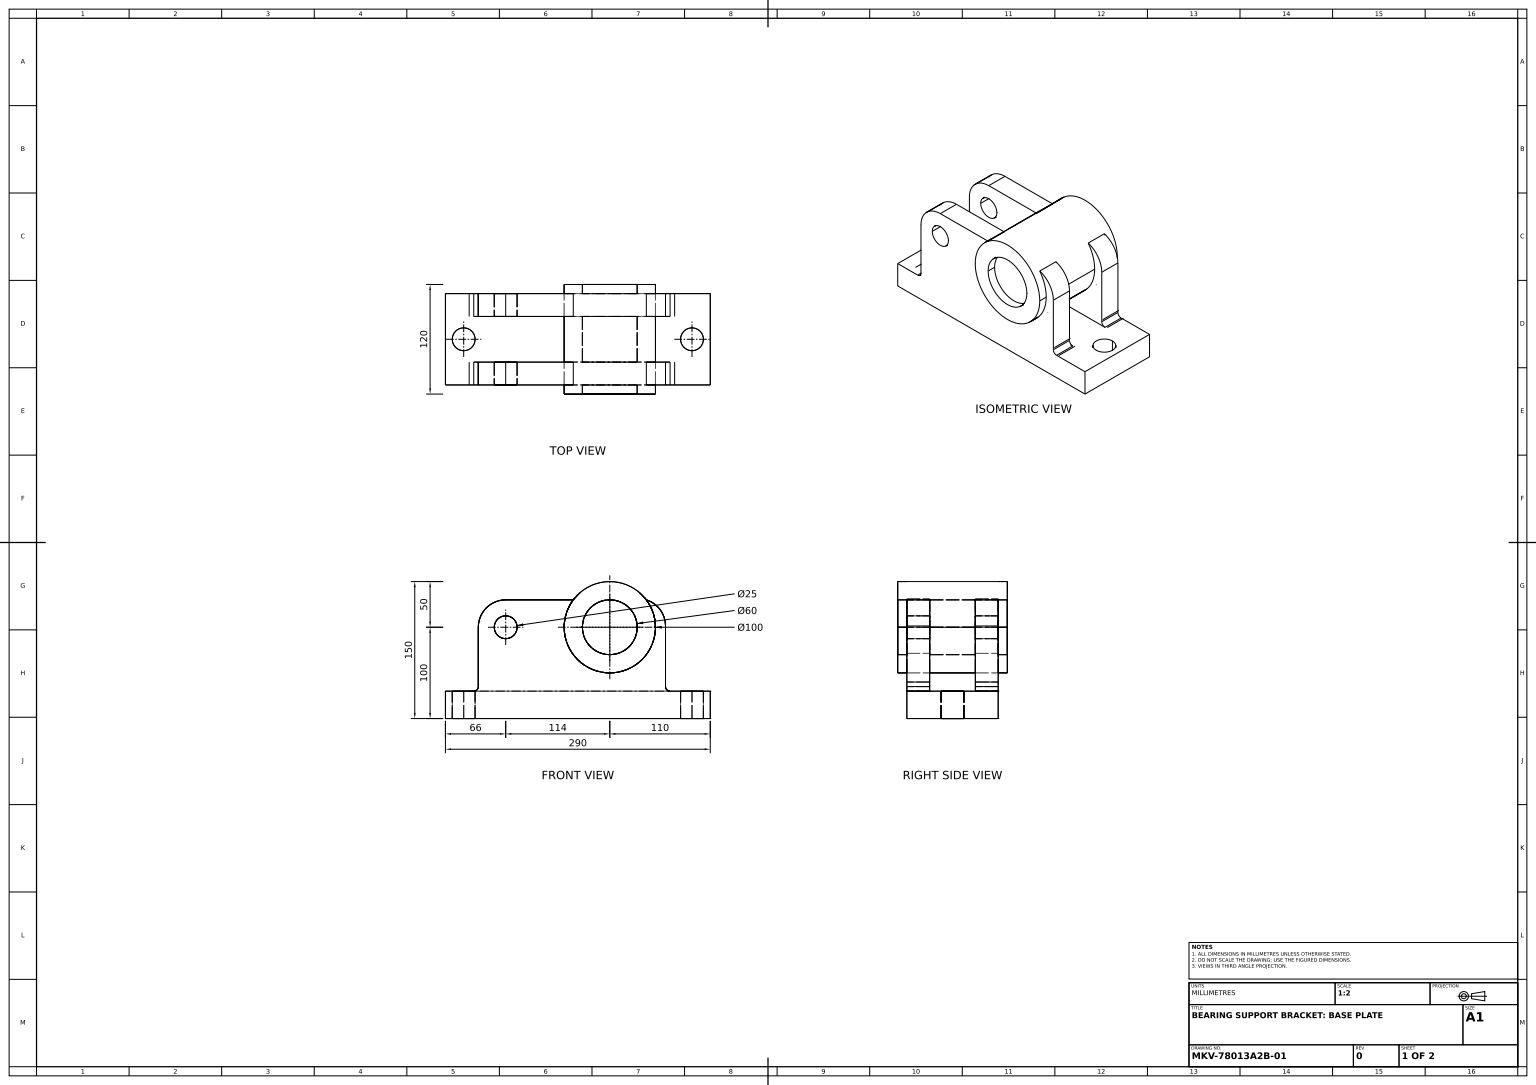
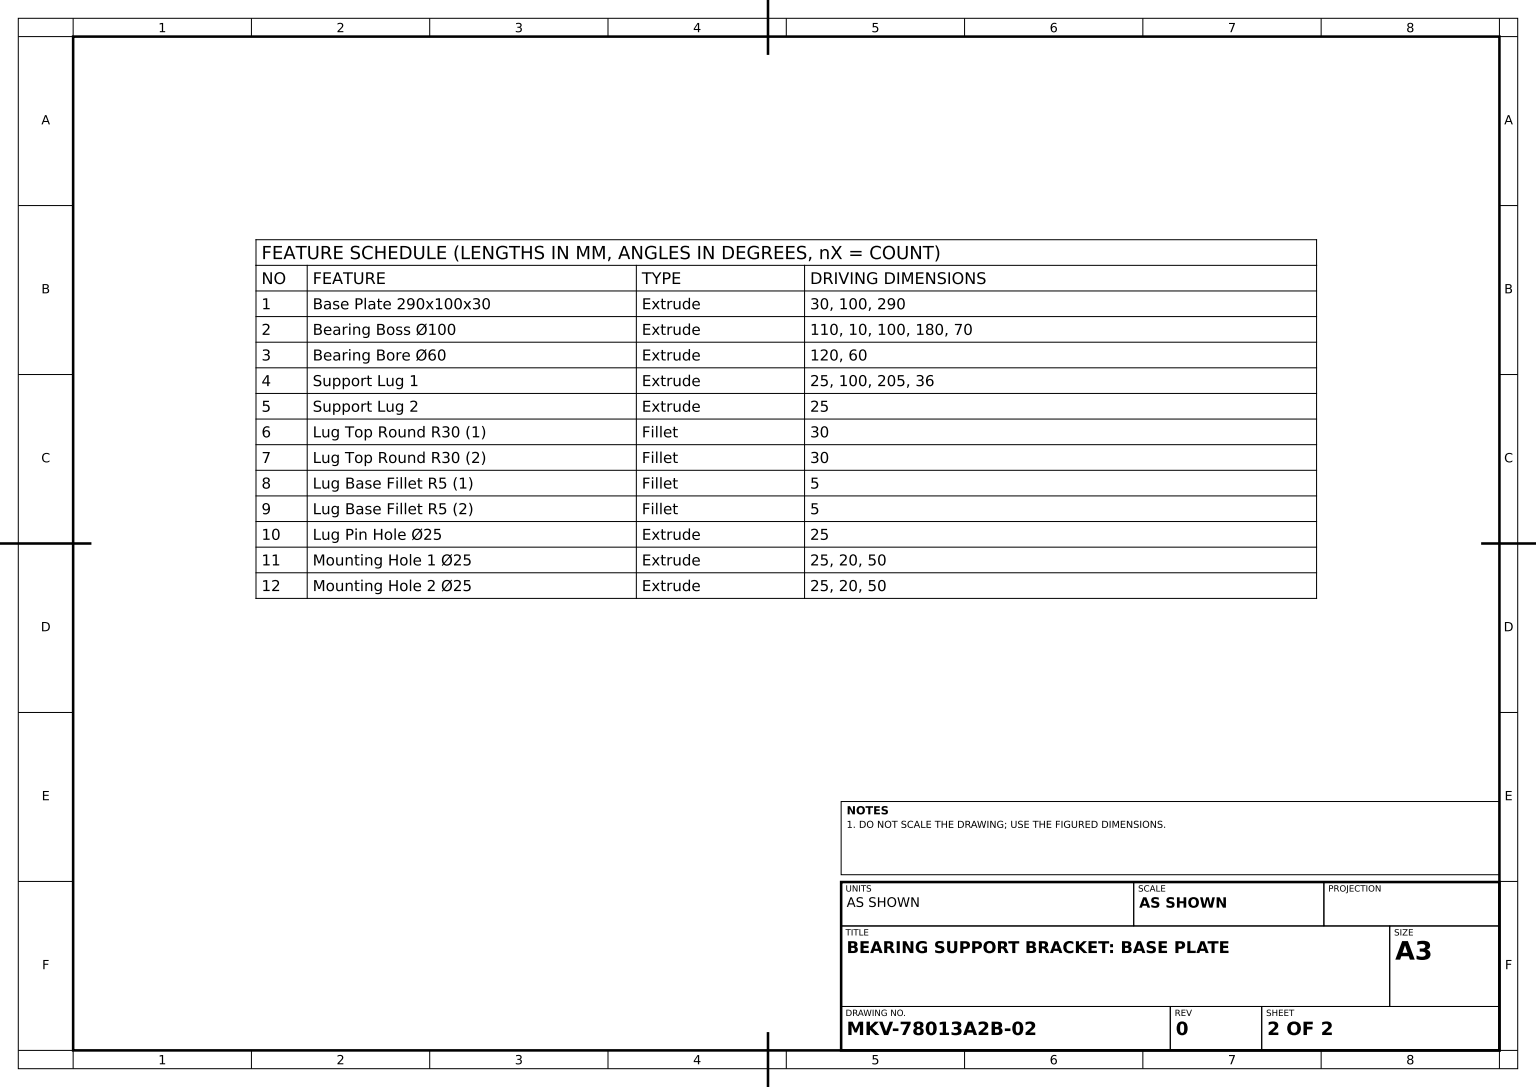
ISO-10303-21;
HEADER;
FILE_DESCRIPTION((''),'2;1');
FILE_NAME('','',(''),(''),'','','');
FILE_SCHEMA(('AUTOMOTIVE_DESIGN'));
ENDSEC;
DATA;
#1=APPLICATION_CONTEXT('');
#2=PRODUCT_CONTEXT('',#1,'mechanical');
#3=PRODUCT('','','',(#2));
#4=PRODUCT_DEFINITION_FORMATION('','',#3);
#5=PRODUCT_DEFINITION_CONTEXT('',#1,'design');
#6=PRODUCT_DEFINITION('','',#4,#5);
#7=PRODUCT_DEFINITION_SHAPE('','',#6);
#8=(LENGTH_UNIT()NAMED_UNIT(*)SI_UNIT(.MILLI.,.METRE.));
#9=(NAMED_UNIT(*)PLANE_ANGLE_UNIT()SI_UNIT($,.RADIAN.));
#10=(NAMED_UNIT(*)SI_UNIT($,.STERADIAN.)SOLID_ANGLE_UNIT());
#11=UNCERTAINTY_MEASURE_WITH_UNIT(LENGTH_MEASURE(1.E-05),#8,'distance_accuracy_value','');
#12=(GEOMETRIC_REPRESENTATION_CONTEXT(3)GLOBAL_UNCERTAINTY_ASSIGNED_CONTEXT((#11))GLOBAL_UNIT_ASSIGNED_CONTEXT((#8,#9,#10))REPRESENTATION_CONTEXT('',''));
#13=CARTESIAN_POINT('',(78.5,100.,-100.));
#14=VERTEX_POINT('',#13);
#15=CARTESIAN_POINT('',(78.5,100.,-75.));
#16=VERTEX_POINT('',#15);
#17=CARTESIAN_POINT('',(78.5,100.,-110.));
#18=DIRECTION('',(0.,0.,1.));
#19=VECTOR('',#18,1000.);
#20=LINE('',#17,#19);
#21=EDGE_CURVE('',#14,#16,#20,.T.);
#22=ORIENTED_EDGE('',*,*,#21,.T.);
#23=CARTESIAN_POINT('',(53.5,100.,-75.));
#24=VERTEX_POINT('',#23);
#25=CARTESIAN_POINT('',(66.,100.,-75.));
#26=DIRECTION('',(1.,0.,0.));
#27=AXIS2_PLACEMENT_3D('',#25,#18,#26);
#28=CIRCLE('',#27,12.5);
#29=EDGE_CURVE('',#16,#24,#28,.T.);
#30=ORIENTED_EDGE('',*,*,#29,.T.);
#31=CARTESIAN_POINT('',(53.5,100.,-100.));
#32=VERTEX_POINT('',#31);
#33=CARTESIAN_POINT('',(53.5,100.,-110.));
#34=LINE('',#33,#19);
#35=EDGE_CURVE('',#32,#24,#34,.T.);
#36=ORIENTED_EDGE('',*,*,#35,.F.);
#37=CARTESIAN_POINT('',(66.,100.,-100.));
#38=AXIS2_PLACEMENT_3D('',#37,#18,#26);
#39=CIRCLE('',#38,12.5);
#40=EDGE_CURVE('',#14,#32,#39,.T.);
#41=ORIENTED_EDGE('',*,*,#40,.F.);
#42=EDGE_LOOP('',(#22,#30,#36,#41));
#43=FACE_OUTER_BOUND('',#42,.T.);
#44=CARTESIAN_POINT('',(66.,100.,-110.));
#45=AXIS2_PLACEMENT_3D('',#44,#18,#26);
#46=CYLINDRICAL_SURFACE('',#45,12.5);
#47=ADVANCED_FACE('',(#43),#46,.F.);
#48=CARTESIAN_POINT('',(36.,100.,-75.));
#49=VERTEX_POINT('',#48);
#50=CARTESIAN_POINT('',(36.,100.,-100.));
#51=VERTEX_POINT('',#50);
#52=DIRECTION('',(0.,0.,-1.));
#53=VECTOR('',#52,1000.);
#54=LINE('',#48,#53);
#55=EDGE_CURVE('',#49,#51,#54,.T.);
#56=ORIENTED_EDGE('',*,*,#55,.T.);
#57=CARTESIAN_POINT('',(36.,35.,-100.));
#58=VERTEX_POINT('',#57);
#59=CARTESIAN_POINT('',(36.,130.,-100.));
#60=DIRECTION('',(0.,1.,0.));
#61=VECTOR('',#60,1000.);
#62=LINE('',#59,#61);
#63=EDGE_CURVE('',#58,#51,#62,.T.);
#64=ORIENTED_EDGE('',*,*,#63,.F.);
#65=CARTESIAN_POINT('',(36.,35.,-75.));
#66=VERTEX_POINT('',#65);
#67=LINE('',#65,#19);
#68=EDGE_CURVE('',#58,#66,#67,.T.);
#69=ORIENTED_EDGE('',*,*,#68,.T.);
#70=CARTESIAN_POINT('',(36.,130.,-75.));
#71=LINE('',#70,#61);
#72=EDGE_CURVE('',#66,#49,#71,.T.);
#73=ORIENTED_EDGE('',*,*,#72,.T.);
#74=EDGE_LOOP('',(#56,#64,#69,#73));
#75=FACE_OUTER_BOUND('',#74,.T.);
#76=DIRECTION('',(-1.,0.,0.));
#77=AXIS2_PLACEMENT_3D('',#70,#76,#18);
#78=PLANE('',#77);
#79=ADVANCED_FACE('',(#75),#78,.T.);
#80=CARTESIAN_POINT('',(210.,100.,-100.));
#81=VERTEX_POINT('',#80);
#82=CARTESIAN_POINT('',(150.,100.,-100.));
#83=VERTEX_POINT('',#82);
#84=CARTESIAN_POINT('',(180.,100.,-100.));
#85=AXIS2_PLACEMENT_3D('',#84,#52,#26);
#86=CIRCLE('',#85,30.);
#87=EDGE_CURVE('',#81,#83,#86,.T.);
#88=ORIENTED_EDGE('',*,*,#87,.T.);
#89=EDGE_CURVE('',#83,#81,#86,.T.);
#90=ORIENTED_EDGE('',*,*,#89,.T.);
#91=EDGE_LOOP('',(#88,#90));
#92=FACE_OUTER_BOUND('',#91,.T.);
#93=CARTESIAN_POINT('',(0.,0.,-100.));
#94=AXIS2_PLACEMENT_3D('',#93,#18,#26);
#95=PLANE('',#94);
#96=ADVANCED_FACE('',(#92),#95,.F.);
#97=ORIENTED_EDGE('',*,*,#68,.F.);
#98=CARTESIAN_POINT('',(31.,30.,-100.));
#99=VERTEX_POINT('',#98);
#100=CARTESIAN_POINT('',(31.,35.,-100.));
#101=AXIS2_PLACEMENT_3D('',#100,#18,#26);
#102=CIRCLE('',#101,5.);
#103=EDGE_CURVE('',#99,#58,#102,.T.);
#104=ORIENTED_EDGE('',*,*,#103,.F.);
#105=CARTESIAN_POINT('',(31.,30.,-75.));
#106=VERTEX_POINT('',#105);
#107=CARTESIAN_POINT('',(31.,30.,0.));
#108=LINE('',#107,#53);
#109=EDGE_CURVE('',#106,#99,#108,.T.);
#110=ORIENTED_EDGE('',*,*,#109,.F.);
#111=CARTESIAN_POINT('',(31.,35.,-75.));
#112=AXIS2_PLACEMENT_3D('',#111,#52,#26);
#113=CIRCLE('',#112,5.);
#114=EDGE_CURVE('',#66,#106,#113,.T.);
#115=ORIENTED_EDGE('',*,*,#114,.F.);
#116=EDGE_LOOP('',(#97,#104,#110,#115));
#117=FACE_OUTER_BOUND('',#116,.T.);
#118=CARTESIAN_POINT('',(31.,35.,0.));
#119=AXIS2_PLACEMENT_3D('',#118,#52,#76);
#120=CYLINDRICAL_SURFACE('',#119,5.);
#121=ADVANCED_FACE('',(#117),#120,.F.);
#122=CARTESIAN_POINT('',(150.,100.,10.));
#123=VERTEX_POINT('',#122);
#124=CARTESIAN_POINT('',(210.,100.,10.));
#125=VERTEX_POINT('',#124);
#126=CARTESIAN_POINT('',(180.,100.,10.));
#127=AXIS2_PLACEMENT_3D('',#126,#18,#26);
#128=CIRCLE('',#127,30.);
#129=EDGE_CURVE('',#123,#125,#128,.T.);
#130=ORIENTED_EDGE('',*,*,#129,.F.);
#131=EDGE_CURVE('',#125,#123,#128,.T.);
#132=ORIENTED_EDGE('',*,*,#131,.F.);
#133=EDGE_LOOP('',(#130,#132));
#134=FACE_BOUND('',#133,.T.);
#135=CARTESIAN_POINT('',(130.,100.,10.));
#136=VERTEX_POINT('',#135);
#137=CARTESIAN_POINT('',(230.,100.,10.));
#138=VERTEX_POINT('',#137);
#139=CIRCLE('',#127,50.);
#140=EDGE_CURVE('',#136,#138,#139,.T.);
#141=ORIENTED_EDGE('',*,*,#140,.T.);
#142=EDGE_CURVE('',#138,#136,#139,.T.);
#143=ORIENTED_EDGE('',*,*,#142,.T.);
#144=EDGE_LOOP('',(#141,#143));
#145=FACE_OUTER_BOUND('',#144,.T.);
#146=PLANE('',#127);
#147=ADVANCED_FACE('',(#134,#145),#146,.T.);
#148=CARTESIAN_POINT('',(290.,0.,0.));
#149=VERTEX_POINT('',#148);
#150=CARTESIAN_POINT('',(290.,0.,-100.));
#151=VERTEX_POINT('',#150);
#152=LINE('',#150,#53);
#153=EDGE_CURVE('',#149,#151,#152,.T.);
#154=ORIENTED_EDGE('',*,*,#153,.T.);
#155=CARTESIAN_POINT('',(290.,30.,-100.));
#156=VERTEX_POINT('',#155);
#157=DIRECTION('',(0.,-1.,0.));
#158=VECTOR('',#157,1000.);
#159=LINE('',#155,#158);
#160=EDGE_CURVE('',#156,#151,#159,.T.);
#161=ORIENTED_EDGE('',*,*,#160,.F.);
#162=CARTESIAN_POINT('',(290.,30.,0.));
#163=VERTEX_POINT('',#162);
#164=LINE('',#155,#53);
#165=EDGE_CURVE('',#163,#156,#164,.T.);
#166=ORIENTED_EDGE('',*,*,#165,.F.);
#167=LINE('',#162,#158);
#168=EDGE_CURVE('',#163,#149,#167,.T.);
#169=ORIENTED_EDGE('',*,*,#168,.T.);
#170=EDGE_LOOP('',(#154,#161,#166,#169));
#171=FACE_OUTER_BOUND('',#170,.T.);
#172=AXIS2_PLACEMENT_3D('',#155,#76,#18);
#173=PLANE('',#172);
#174=ADVANCED_FACE('',(#171),#173,.F.);
#175=CARTESIAN_POINT('',(230.,100.,0.));
#176=VERTEX_POINT('',#175);
#177=LINE('',#137,#53);
#178=EDGE_CURVE('',#138,#176,#177,.T.);
#179=ORIENTED_EDGE('',*,*,#178,.F.);
#180=ORIENTED_EDGE('',*,*,#140,.F.);
#181=CARTESIAN_POINT('',(130.,100.,0.));
#182=VERTEX_POINT('',#181);
#183=LINE('',#135,#53);
#184=EDGE_CURVE('',#136,#182,#183,.T.);
#185=ORIENTED_EDGE('',*,*,#184,.T.);
#186=CARTESIAN_POINT('',(180.,100.,0.));
#187=AXIS2_PLACEMENT_3D('',#186,#18,#76);
#188=CIRCLE('',#187,50.);
#189=EDGE_CURVE('',#182,#176,#188,.T.);
#190=ORIENTED_EDGE('',*,*,#189,.T.);
#191=EDGE_LOOP('',(#179,#180,#185,#190));
#192=FACE_OUTER_BOUND('',#191,.T.);
#193=AXIS2_PLACEMENT_3D('',#126,#52,#76);
#194=CYLINDRICAL_SURFACE('',#193,50.);
#195=ADVANCED_FACE('',(#192),#194,.T.);
#196=CARTESIAN_POINT('',(53.5,100.,-25.));
#197=VERTEX_POINT('',#196);
#198=CARTESIAN_POINT('',(78.5,100.,-25.));
#199=VERTEX_POINT('',#198);
#200=CARTESIAN_POINT('',(66.,100.,-25.));
#201=AXIS2_PLACEMENT_3D('',#200,#52,#76);
#202=CIRCLE('',#201,12.5);
#203=EDGE_CURVE('',#197,#199,#202,.T.);
#204=ORIENTED_EDGE('',*,*,#203,.T.);
#205=CARTESIAN_POINT('',(78.5,100.,0.));
#206=VERTEX_POINT('',#205);
#207=EDGE_CURVE('',#199,#206,#20,.T.);
#208=ORIENTED_EDGE('',*,*,#207,.T.);
#209=CARTESIAN_POINT('',(53.5,100.,0.));
#210=VERTEX_POINT('',#209);
#211=CARTESIAN_POINT('',(66.,100.,0.));
#212=AXIS2_PLACEMENT_3D('',#211,#18,#26);
#213=CIRCLE('',#212,12.5);
#214=EDGE_CURVE('',#206,#210,#213,.T.);
#215=ORIENTED_EDGE('',*,*,#214,.T.);
#216=EDGE_CURVE('',#197,#210,#34,.T.);
#217=ORIENTED_EDGE('',*,*,#216,.F.);
#218=EDGE_LOOP('',(#204,#208,#215,#217));
#219=FACE_OUTER_BOUND('',#218,.T.);
#220=ADVANCED_FACE('',(#219),#46,.F.);
#221=CARTESIAN_POINT('',(230.,100.,-110.));
#222=VERTEX_POINT('',#221);
#223=CARTESIAN_POINT('',(130.,100.,-110.));
#224=VERTEX_POINT('',#223);
#225=CARTESIAN_POINT('',(180.,100.,-110.));
#226=AXIS2_PLACEMENT_3D('',#225,#18,#26);
#227=CIRCLE('',#226,50.);
#228=EDGE_CURVE('',#222,#224,#227,.T.);
#229=ORIENTED_EDGE('',*,*,#228,.F.);
#230=EDGE_CURVE('',#224,#222,#227,.T.);
#231=ORIENTED_EDGE('',*,*,#230,.F.);
#232=EDGE_LOOP('',(#229,#231));
#233=FACE_OUTER_BOUND('',#232,.T.);
#234=CARTESIAN_POINT('',(210.,100.,-110.));
#235=VERTEX_POINT('',#234);
#236=CARTESIAN_POINT('',(150.,100.,-110.));
#237=VERTEX_POINT('',#236);
#238=CIRCLE('',#226,30.);
#239=EDGE_CURVE('',#235,#237,#238,.T.);
#240=ORIENTED_EDGE('',*,*,#239,.T.);
#241=EDGE_CURVE('',#237,#235,#238,.T.);
#242=ORIENTED_EDGE('',*,*,#241,.T.);
#243=EDGE_LOOP('',(#240,#242));
#244=FACE_BOUND('',#243,.T.);
#245=PLANE('',#226);
#246=ADVANCED_FACE('',(#233,#244),#245,.F.);
#247=CARTESIAN_POINT('',(270.,0.,-62.5));
#248=VERTEX_POINT('',#247);
#249=CARTESIAN_POINT('',(270.,0.,-37.5));
#250=VERTEX_POINT('',#249);
#251=CARTESIAN_POINT('',(270.,0.,-50.));
#252=AXIS2_PLACEMENT_3D('',#251,#60,#18);
#253=CIRCLE('',#252,12.5);
#254=EDGE_CURVE('',#248,#250,#253,.T.);
#255=ORIENTED_EDGE('',*,*,#254,.T.);
#256=EDGE_CURVE('',#250,#248,#253,.T.);
#257=ORIENTED_EDGE('',*,*,#256,.T.);
#258=EDGE_LOOP('',(#255,#257));
#259=FACE_BOUND('',#258,.T.);
#260=CARTESIAN_POINT('',(20.,0.,-37.5));
#261=VERTEX_POINT('',#260);
#262=CARTESIAN_POINT('',(20.,0.,-62.5));
#263=VERTEX_POINT('',#262);
#264=CARTESIAN_POINT('',(20.,0.,-50.));
#265=AXIS2_PLACEMENT_3D('',#264,#60,#18);
#266=CIRCLE('',#265,12.5);
#267=EDGE_CURVE('',#261,#263,#266,.T.);
#268=ORIENTED_EDGE('',*,*,#267,.T.);
#269=EDGE_CURVE('',#263,#261,#266,.T.);
#270=ORIENTED_EDGE('',*,*,#269,.T.);
#271=EDGE_LOOP('',(#268,#270));
#272=FACE_BOUND('',#271,.T.);
#273=CARTESIAN_POINT('',(0.,0.,0.));
#274=VERTEX_POINT('',#273);
#275=VECTOR('',#26,1000.);
#276=LINE('',#148,#275);
#277=EDGE_CURVE('',#274,#149,#276,.T.);
#278=ORIENTED_EDGE('',*,*,#277,.F.);
#279=VERTEX_POINT('',#93);
#280=LINE('',#273,#19);
#281=EDGE_CURVE('',#279,#274,#280,.T.);
#282=ORIENTED_EDGE('',*,*,#281,.F.);
#283=VECTOR('',#76,1000.);
#284=LINE('',#93,#283);
#285=EDGE_CURVE('',#151,#279,#284,.T.);
#286=ORIENTED_EDGE('',*,*,#285,.F.);
#287=ORIENTED_EDGE('',*,*,#153,.F.);
#288=EDGE_LOOP('',(#278,#282,#286,#287));
#289=FACE_OUTER_BOUND('',#288,.T.);
#290=AXIS2_PLACEMENT_3D('',#273,#157,#52);
#291=PLANE('',#290);
#292=ADVANCED_FACE('',(#259,#272,#289),#291,.T.);
#293=CARTESIAN_POINT('',(66.,130.,-25.));
#294=VERTEX_POINT('',#293);
#295=CARTESIAN_POINT('',(66.,130.,0.));
#296=VERTEX_POINT('',#295);
#297=LINE('',#293,#19);
#298=EDGE_CURVE('',#294,#296,#297,.T.);
#299=ORIENTED_EDGE('',*,*,#298,.T.);
#300=CARTESIAN_POINT('',(140.,130.,0.));
#301=VERTEX_POINT('',#300);
#302=CARTESIAN_POINT('',(36.,130.,0.));
#303=LINE('',#302,#283);
#304=EDGE_CURVE('',#301,#296,#303,.T.);
#305=ORIENTED_EDGE('',*,*,#304,.F.);
#306=CARTESIAN_POINT('',(140.,130.,-25.));
#307=VERTEX_POINT('',#306);
#308=CARTESIAN_POINT('',(140.,130.,10.));
#309=LINE('',#308,#53);
#310=EDGE_CURVE('',#301,#307,#309,.T.);
#311=ORIENTED_EDGE('',*,*,#310,.T.);
#312=CARTESIAN_POINT('',(36.,130.,-25.));
#313=LINE('',#312,#283);
#314=EDGE_CURVE('',#307,#294,#313,.T.);
#315=ORIENTED_EDGE('',*,*,#314,.T.);
#316=EDGE_LOOP('',(#299,#305,#311,#315));
#317=FACE_OUTER_BOUND('',#316,.T.);
#318=AXIS2_PLACEMENT_3D('',#312,#60,#18);
#319=PLANE('',#318);
#320=ADVANCED_FACE('',(#317),#319,.T.);
#321=ORIENTED_EDGE('',*,*,#35,.T.);
#322=EDGE_CURVE('',#24,#16,#28,.T.);
#323=ORIENTED_EDGE('',*,*,#322,.T.);
#324=ORIENTED_EDGE('',*,*,#21,.F.);
#325=EDGE_CURVE('',#32,#14,#39,.T.);
#326=ORIENTED_EDGE('',*,*,#325,.F.);
#327=EDGE_LOOP('',(#321,#323,#324,#326));
#328=FACE_OUTER_BOUND('',#327,.T.);
#329=ADVANCED_FACE('',(#328),#46,.F.);
#330=CARTESIAN_POINT('',(36.,100.,0.));
#331=VERTEX_POINT('',#330);
#332=CARTESIAN_POINT('',(36.,100.,-25.));
#333=VERTEX_POINT('',#332);
#334=LINE('',#332,#53);
#335=EDGE_CURVE('',#331,#333,#334,.T.);
#336=ORIENTED_EDGE('',*,*,#335,.F.);
#337=AXIS2_PLACEMENT_3D('',#211,#18,#76);
#338=CIRCLE('',#337,30.);
#339=EDGE_CURVE('',#296,#331,#338,.T.);
#340=ORIENTED_EDGE('',*,*,#339,.F.);
#341=ORIENTED_EDGE('',*,*,#298,.F.);
#342=CIRCLE('',#201,30.);
#343=EDGE_CURVE('',#333,#294,#342,.T.);
#344=ORIENTED_EDGE('',*,*,#343,.F.);
#345=EDGE_LOOP('',(#336,#340,#341,#344));
#346=FACE_OUTER_BOUND('',#345,.T.);
#347=AXIS2_PLACEMENT_3D('',#200,#18,#26);
#348=CYLINDRICAL_SURFACE('',#347,30.);
#349=ADVANCED_FACE('',(#346),#348,.T.);
#350=CARTESIAN_POINT('',(130.,100.,-100.));
#351=VERTEX_POINT('',#350);
#352=CARTESIAN_POINT('',(230.,100.,-100.));
#353=VERTEX_POINT('',#352);
#354=AXIS2_PLACEMENT_3D('',#84,#18,#26);
#355=CIRCLE('',#354,50.);
#356=EDGE_CURVE('',#351,#353,#355,.T.);
#357=ORIENTED_EDGE('',*,*,#356,.F.);
#358=EDGE_CURVE('',#351,#224,#183,.T.);
#359=ORIENTED_EDGE('',*,*,#358,.T.);
#360=ORIENTED_EDGE('',*,*,#230,.T.);
#361=EDGE_CURVE('',#353,#222,#177,.T.);
#362=ORIENTED_EDGE('',*,*,#361,.F.);
#363=EDGE_LOOP('',(#357,#359,#360,#362));
#364=FACE_OUTER_BOUND('',#363,.T.);
#365=ADVANCED_FACE('',(#364),#194,.T.);
#366=ORIENTED_EDGE('',*,*,#40,.T.);
#367=ORIENTED_EDGE('',*,*,#325,.T.);
#368=EDGE_LOOP('',(#366,#367));
#369=FACE_BOUND('',#368,.T.);
#370=CARTESIAN_POINT('',(220.,130.,-100.));
#371=VERTEX_POINT('',#370);
#372=CARTESIAN_POINT('',(241.,101.381824,-100.));
#373=VERTEX_POINT('',#372);
#374=CARTESIAN_POINT('',(211.,101.381824,-100.));
#375=AXIS2_PLACEMENT_3D('',#374,#52,#26);
#376=CIRCLE('',#375,30.);
#377=EDGE_CURVE('',#371,#373,#376,.T.);
#378=ORIENTED_EDGE('',*,*,#377,.T.);
#379=CARTESIAN_POINT('',(241.,35.,-100.));
#380=VERTEX_POINT('',#379);
#381=CARTESIAN_POINT('',(241.,30.,-100.));
#382=LINE('',#381,#158);
#383=EDGE_CURVE('',#373,#380,#382,.T.);
#384=ORIENTED_EDGE('',*,*,#383,.T.);
#385=CARTESIAN_POINT('',(246.,30.,-100.));
#386=VERTEX_POINT('',#385);
#387=CARTESIAN_POINT('',(246.,35.,-100.));
#388=AXIS2_PLACEMENT_3D('',#387,#18,#26);
#389=CIRCLE('',#388,5.);
#390=EDGE_CURVE('',#380,#386,#389,.T.);
#391=ORIENTED_EDGE('',*,*,#390,.T.);
#392=CARTESIAN_POINT('',(0.,30.,-100.));
#393=LINE('',#392,#283);
#394=EDGE_CURVE('',#156,#386,#393,.T.);
#395=ORIENTED_EDGE('',*,*,#394,.F.);
#396=ORIENTED_EDGE('',*,*,#160,.T.);
#397=ORIENTED_EDGE('',*,*,#285,.T.);
#398=VERTEX_POINT('',#392);
#399=LINE('',#392,#158);
#400=EDGE_CURVE('',#398,#279,#399,.T.);
#401=ORIENTED_EDGE('',*,*,#400,.F.);
#402=EDGE_CURVE('',#99,#398,#393,.T.);
#403=ORIENTED_EDGE('',*,*,#402,.F.);
#404=ORIENTED_EDGE('',*,*,#103,.T.);
#405=ORIENTED_EDGE('',*,*,#63,.T.);
#406=CARTESIAN_POINT('',(66.,130.,-100.));
#407=VERTEX_POINT('',#406);
#408=AXIS2_PLACEMENT_3D('',#37,#52,#26);
#409=CIRCLE('',#408,30.);
#410=EDGE_CURVE('',#51,#407,#409,.T.);
#411=ORIENTED_EDGE('',*,*,#410,.T.);
#412=CARTESIAN_POINT('',(140.,130.,-100.));
#413=VERTEX_POINT('',#412);
#414=CARTESIAN_POINT('',(241.,130.,-100.));
#415=LINE('',#414,#275);
#416=EDGE_CURVE('',#407,#413,#415,.T.);
#417=ORIENTED_EDGE('',*,*,#416,.T.);
#418=EDGE_CURVE('',#413,#351,#355,.T.);
#419=ORIENTED_EDGE('',*,*,#418,.T.);
#420=ORIENTED_EDGE('',*,*,#356,.T.);
#421=EDGE_CURVE('',#353,#371,#355,.T.);
#422=ORIENTED_EDGE('',*,*,#421,.T.);
#423=EDGE_LOOP('',(#378,#384,#391,#395,#396,#397,#401,#403,#404,#405,#411,#417,#419,#420,#422));
#424=FACE_OUTER_BOUND('',#423,.T.);
#425=AXIS2_PLACEMENT_3D('',#392,#18,#26);
#426=PLANE('',#425);
#427=ADVANCED_FACE('',(#369,#424),#426,.F.);
#428=CARTESIAN_POINT('',(20.,30.,-62.5));
#429=VERTEX_POINT('',#428);
#430=LINE('',#262,#61);
#431=EDGE_CURVE('',#263,#429,#430,.T.);
#432=ORIENTED_EDGE('',*,*,#431,.F.);
#433=ORIENTED_EDGE('',*,*,#267,.F.);
#434=CARTESIAN_POINT('',(20.,30.,-37.5));
#435=VERTEX_POINT('',#434);
#436=LINE('',#260,#61);
#437=EDGE_CURVE('',#261,#435,#436,.T.);
#438=ORIENTED_EDGE('',*,*,#437,.T.);
#439=CARTESIAN_POINT('',(20.,30.,-50.));
#440=AXIS2_PLACEMENT_3D('',#439,#60,#18);
#441=CIRCLE('',#440,12.5);
#442=EDGE_CURVE('',#435,#429,#441,.T.);
#443=ORIENTED_EDGE('',*,*,#442,.T.);
#444=EDGE_LOOP('',(#432,#433,#438,#443));
#445=FACE_OUTER_BOUND('',#444,.T.);
#446=CYLINDRICAL_SURFACE('',#265,12.5);
#447=ADVANCED_FACE('',(#445),#446,.F.);
#448=CARTESIAN_POINT('',(150.,100.,0.));
#449=VERTEX_POINT('',#448);
#450=CARTESIAN_POINT('',(210.,100.,0.));
#451=VERTEX_POINT('',#450);
#452=AXIS2_PLACEMENT_3D('',#186,#52,#76);
#453=CIRCLE('',#452,30.);
#454=EDGE_CURVE('',#449,#451,#453,.T.);
#455=ORIENTED_EDGE('',*,*,#454,.F.);
#456=EDGE_CURVE('',#451,#449,#453,.T.);
#457=ORIENTED_EDGE('',*,*,#456,.F.);
#458=EDGE_LOOP('',(#455,#457));
#459=FACE_OUTER_BOUND('',#458,.T.);
#460=AXIS2_PLACEMENT_3D('',#162,#52,#76);
#461=PLANE('',#460);
#462=ADVANCED_FACE('',(#459),#461,.F.);
#463=EDGE_CURVE('',#210,#206,#213,.T.);
#464=ORIENTED_EDGE('',*,*,#463,.F.);
#465=ORIENTED_EDGE('',*,*,#214,.F.);
#466=EDGE_LOOP('',(#464,#465));
#467=FACE_BOUND('',#466,.T.);
#468=ORIENTED_EDGE('',*,*,#277,.T.);
#469=ORIENTED_EDGE('',*,*,#168,.F.);
#470=CARTESIAN_POINT('',(246.,30.,0.));
#471=VERTEX_POINT('',#470);
#472=LINE('',#162,#275);
#473=EDGE_CURVE('',#471,#163,#472,.T.);
#474=ORIENTED_EDGE('',*,*,#473,.F.);
#475=CARTESIAN_POINT('',(241.,35.,0.));
#476=VERTEX_POINT('',#475);
#477=CARTESIAN_POINT('',(246.,35.,0.));
#478=AXIS2_PLACEMENT_3D('',#477,#52,#76);
#479=CIRCLE('',#478,5.);
#480=EDGE_CURVE('',#471,#476,#479,.T.);
#481=ORIENTED_EDGE('',*,*,#480,.T.);
#482=CARTESIAN_POINT('',(241.,101.381824,0.));
#483=VERTEX_POINT('',#482);
#484=CARTESIAN_POINT('',(241.,130.,0.));
#485=LINE('',#484,#61);
#486=EDGE_CURVE('',#476,#483,#485,.T.);
#487=ORIENTED_EDGE('',*,*,#486,.T.);
#488=CARTESIAN_POINT('',(220.,130.,0.));
#489=VERTEX_POINT('',#488);
#490=CARTESIAN_POINT('',(211.,101.381824,0.));
#491=AXIS2_PLACEMENT_3D('',#490,#18,#76);
#492=CIRCLE('',#491,30.);
#493=EDGE_CURVE('',#483,#489,#492,.T.);
#494=ORIENTED_EDGE('',*,*,#493,.T.);
#495=EDGE_CURVE('',#176,#489,#188,.T.);
#496=ORIENTED_EDGE('',*,*,#495,.F.);
#497=ORIENTED_EDGE('',*,*,#189,.F.);
#498=EDGE_CURVE('',#301,#182,#188,.T.);
#499=ORIENTED_EDGE('',*,*,#498,.F.);
#500=ORIENTED_EDGE('',*,*,#304,.T.);
#501=ORIENTED_EDGE('',*,*,#339,.T.);
#502=CARTESIAN_POINT('',(36.,35.,0.));
#503=VERTEX_POINT('',#502);
#504=CARTESIAN_POINT('',(36.,30.,0.));
#505=LINE('',#504,#158);
#506=EDGE_CURVE('',#331,#503,#505,.T.);
#507=ORIENTED_EDGE('',*,*,#506,.T.);
#508=VERTEX_POINT('',#107);
#509=CIRCLE('',#119,5.);
#510=EDGE_CURVE('',#503,#508,#509,.T.);
#511=ORIENTED_EDGE('',*,*,#510,.T.);
#512=CARTESIAN_POINT('',(0.,30.,0.));
#513=VERTEX_POINT('',#512);
#514=EDGE_CURVE('',#513,#508,#472,.T.);
#515=ORIENTED_EDGE('',*,*,#514,.F.);
#516=LINE('',#512,#158);
#517=EDGE_CURVE('',#513,#274,#516,.T.);
#518=ORIENTED_EDGE('',*,*,#517,.T.);
#519=EDGE_LOOP('',(#468,#469,#474,#481,#487,#494,#496,#497,#499,#500,#501,#507,#511,#515,#518));
#520=FACE_OUTER_BOUND('',#519,.T.);
#521=ADVANCED_FACE('',(#467,#520),#461,.F.);
#522=CARTESIAN_POINT('',(270.,30.,-62.5));
#523=VERTEX_POINT('',#522);
#524=LINE('',#247,#61);
#525=EDGE_CURVE('',#248,#523,#524,.T.);
#526=ORIENTED_EDGE('',*,*,#525,.F.);
#527=ORIENTED_EDGE('',*,*,#256,.F.);
#528=CARTESIAN_POINT('',(270.,30.,-37.5));
#529=VERTEX_POINT('',#528);
#530=LINE('',#249,#61);
#531=EDGE_CURVE('',#250,#529,#530,.T.);
#532=ORIENTED_EDGE('',*,*,#531,.T.);
#533=CARTESIAN_POINT('',(270.,30.,-50.));
#534=AXIS2_PLACEMENT_3D('',#533,#60,#18);
#535=CIRCLE('',#534,12.5);
#536=EDGE_CURVE('',#529,#523,#535,.T.);
#537=ORIENTED_EDGE('',*,*,#536,.T.);
#538=EDGE_LOOP('',(#526,#527,#532,#537));
#539=FACE_OUTER_BOUND('',#538,.T.);
#540=CYLINDRICAL_SURFACE('',#252,12.5);
#541=ADVANCED_FACE('',(#539),#540,.F.);
#542=ORIENTED_EDGE('',*,*,#241,.F.);
#543=LINE('',#236,#19);
#544=EDGE_CURVE('',#237,#83,#543,.T.);
#545=ORIENTED_EDGE('',*,*,#544,.T.);
#546=ORIENTED_EDGE('',*,*,#87,.F.);
#547=LINE('',#234,#19);
#548=EDGE_CURVE('',#235,#81,#547,.T.);
#549=ORIENTED_EDGE('',*,*,#548,.F.);
#550=EDGE_LOOP('',(#542,#545,#546,#549));
#551=FACE_OUTER_BOUND('',#550,.T.);
#552=CYLINDRICAL_SURFACE('',#226,30.);
#553=ADVANCED_FACE('',(#551),#552,.F.);
#554=ORIENTED_EDGE('',*,*,#207,.F.);
#555=EDGE_CURVE('',#199,#197,#202,.T.);
#556=ORIENTED_EDGE('',*,*,#555,.T.);
#557=ORIENTED_EDGE('',*,*,#216,.T.);
#558=ORIENTED_EDGE('',*,*,#463,.T.);
#559=EDGE_LOOP('',(#554,#556,#557,#558));
#560=FACE_OUTER_BOUND('',#559,.T.);
#561=ADVANCED_FACE('',(#560),#46,.F.);
#562=CARTESIAN_POINT('',(246.,30.,-75.));
#563=VERTEX_POINT('',#562);
#564=CARTESIAN_POINT('',(241.,35.,-75.));
#565=VERTEX_POINT('',#564);
#566=CARTESIAN_POINT('',(246.,35.,-75.));
#567=AXIS2_PLACEMENT_3D('',#566,#52,#26);
#568=CIRCLE('',#567,5.);
#569=EDGE_CURVE('',#563,#565,#568,.T.);
#570=ORIENTED_EDGE('',*,*,#569,.F.);
#571=LINE('',#470,#19);
#572=EDGE_CURVE('',#386,#563,#571,.T.);
#573=ORIENTED_EDGE('',*,*,#572,.F.);
#574=ORIENTED_EDGE('',*,*,#390,.F.);
#575=LINE('',#564,#53);
#576=EDGE_CURVE('',#565,#380,#575,.T.);
#577=ORIENTED_EDGE('',*,*,#576,.F.);
#578=EDGE_LOOP('',(#570,#573,#574,#577));
#579=FACE_OUTER_BOUND('',#578,.T.);
#580=AXIS2_PLACEMENT_3D('',#566,#52,#76);
#581=CYLINDRICAL_SURFACE('',#580,5.);
#582=ADVANCED_FACE('',(#579),#581,.F.);
#583=ORIENTED_EDGE('',*,*,#456,.T.);
#584=EDGE_CURVE('',#449,#123,#543,.T.);
#585=ORIENTED_EDGE('',*,*,#584,.T.);
#586=ORIENTED_EDGE('',*,*,#129,.T.);
#587=EDGE_CURVE('',#451,#125,#547,.T.);
#588=ORIENTED_EDGE('',*,*,#587,.F.);
#589=EDGE_LOOP('',(#583,#585,#586,#588));
#590=FACE_OUTER_BOUND('',#589,.T.);
#591=ADVANCED_FACE('',(#590),#552,.F.);
#592=CARTESIAN_POINT('',(130.,100.,-25.));
#593=VERTEX_POINT('',#592);
#594=CARTESIAN_POINT('',(230.,100.,-25.));
#595=VERTEX_POINT('',#594);
#596=CARTESIAN_POINT('',(180.,100.,-25.));
#597=AXIS2_PLACEMENT_3D('',#596,#18,#76);
#598=CIRCLE('',#597,50.);
#599=EDGE_CURVE('',#593,#595,#598,.T.);
#600=ORIENTED_EDGE('',*,*,#599,.F.);
#601=CARTESIAN_POINT('',(130.,100.,-75.));
#602=VERTEX_POINT('',#601);
#603=EDGE_CURVE('',#593,#602,#183,.T.);
#604=ORIENTED_EDGE('',*,*,#603,.T.);
#605=CARTESIAN_POINT('',(230.,100.,-75.));
#606=VERTEX_POINT('',#605);
#607=CARTESIAN_POINT('',(180.,100.,-75.));
#608=AXIS2_PLACEMENT_3D('',#607,#18,#26);
#609=CIRCLE('',#608,50.);
#610=EDGE_CURVE('',#602,#606,#609,.T.);
#611=ORIENTED_EDGE('',*,*,#610,.T.);
#612=EDGE_CURVE('',#595,#606,#177,.T.);
#613=ORIENTED_EDGE('',*,*,#612,.F.);
#614=EDGE_LOOP('',(#600,#604,#611,#613));
#615=FACE_OUTER_BOUND('',#614,.T.);
#616=ADVANCED_FACE('',(#615),#194,.T.);
#617=CARTESIAN_POINT('',(31.,30.,-25.));
#618=VERTEX_POINT('',#617);
#619=EDGE_CURVE('',#508,#618,#108,.T.);
#620=ORIENTED_EDGE('',*,*,#619,.F.);
#621=ORIENTED_EDGE('',*,*,#510,.F.);
#622=CARTESIAN_POINT('',(36.,35.,-25.));
#623=VERTEX_POINT('',#622);
#624=LINE('',#622,#19);
#625=EDGE_CURVE('',#623,#503,#624,.T.);
#626=ORIENTED_EDGE('',*,*,#625,.F.);
#627=CARTESIAN_POINT('',(31.,35.,-25.));
#628=AXIS2_PLACEMENT_3D('',#627,#18,#76);
#629=CIRCLE('',#628,5.);
#630=EDGE_CURVE('',#618,#623,#629,.T.);
#631=ORIENTED_EDGE('',*,*,#630,.F.);
#632=EDGE_LOOP('',(#620,#621,#626,#631));
#633=FACE_OUTER_BOUND('',#632,.T.);
#634=AXIS2_PLACEMENT_3D('',#627,#18,#26);
#635=CYLINDRICAL_SURFACE('',#634,5.);
#636=ADVANCED_FACE('',(#633),#635,.F.);
#637=ORIENTED_EDGE('',*,*,#203,.F.);
#638=ORIENTED_EDGE('',*,*,#555,.F.);
#639=EDGE_LOOP('',(#637,#638));
#640=FACE_BOUND('',#639,.T.);
#641=ORIENTED_EDGE('',*,*,#314,.F.);
#642=EDGE_CURVE('',#307,#593,#598,.T.);
#643=ORIENTED_EDGE('',*,*,#642,.T.);
#644=ORIENTED_EDGE('',*,*,#599,.T.);
#645=CARTESIAN_POINT('',(220.,130.,-25.));
#646=VERTEX_POINT('',#645);
#647=EDGE_CURVE('',#595,#646,#598,.T.);
#648=ORIENTED_EDGE('',*,*,#647,.T.);
#649=CARTESIAN_POINT('',(241.,101.381824,-25.));
#650=VERTEX_POINT('',#649);
#651=CARTESIAN_POINT('',(211.,101.381824,-25.));
#652=AXIS2_PLACEMENT_3D('',#651,#52,#76);
#653=CIRCLE('',#652,30.);
#654=EDGE_CURVE('',#646,#650,#653,.T.);
#655=ORIENTED_EDGE('',*,*,#654,.T.);
#656=CARTESIAN_POINT('',(241.,35.,-25.));
#657=VERTEX_POINT('',#656);
#658=CARTESIAN_POINT('',(241.,130.,-25.));
#659=LINE('',#658,#61);
#660=EDGE_CURVE('',#657,#650,#659,.T.);
#661=ORIENTED_EDGE('',*,*,#660,.F.);
#662=CARTESIAN_POINT('',(246.,30.,-25.));
#663=VERTEX_POINT('',#662);
#664=CARTESIAN_POINT('',(246.,35.,-25.));
#665=AXIS2_PLACEMENT_3D('',#664,#18,#76);
#666=CIRCLE('',#665,5.);
#667=EDGE_CURVE('',#657,#663,#666,.T.);
#668=ORIENTED_EDGE('',*,*,#667,.T.);
#669=CARTESIAN_POINT('',(241.,30.,-25.));
#670=LINE('',#669,#275);
#671=EDGE_CURVE('',#618,#663,#670,.T.);
#672=ORIENTED_EDGE('',*,*,#671,.F.);
#673=ORIENTED_EDGE('',*,*,#630,.T.);
#674=CARTESIAN_POINT('',(36.,30.,-25.));
#675=LINE('',#674,#158);
#676=EDGE_CURVE('',#333,#623,#675,.T.);
#677=ORIENTED_EDGE('',*,*,#676,.F.);
#678=ORIENTED_EDGE('',*,*,#343,.T.);
#679=EDGE_LOOP('',(#641,#643,#644,#648,#655,#661,#668,#672,#673,#677,#678));
#680=FACE_OUTER_BOUND('',#679,.T.);
#681=CARTESIAN_POINT('',(0.,0.,-25.));
#682=AXIS2_PLACEMENT_3D('',#681,#52,#76);
#683=PLANE('',#682);
#684=ADVANCED_FACE('',(#640,#680),#683,.T.);
#685=ORIENTED_EDGE('',*,*,#544,.F.);
#686=ORIENTED_EDGE('',*,*,#239,.F.);
#687=ORIENTED_EDGE('',*,*,#548,.T.);
#688=ORIENTED_EDGE('',*,*,#89,.F.);
#689=EDGE_LOOP('',(#685,#686,#687,#688));
#690=FACE_OUTER_BOUND('',#689,.T.);
#691=ADVANCED_FACE('',(#690),#552,.F.);
#692=ORIENTED_EDGE('',*,*,#572,.T.);
#693=CARTESIAN_POINT('',(36.,30.,-75.));
#694=LINE('',#693,#283);
#695=EDGE_CURVE('',#563,#106,#694,.T.);
#696=ORIENTED_EDGE('',*,*,#695,.T.);
#697=ORIENTED_EDGE('',*,*,#109,.T.);
#698=ORIENTED_EDGE('',*,*,#402,.T.);
#699=LINE('',#512,#19);
#700=EDGE_CURVE('',#398,#513,#699,.T.);
#701=ORIENTED_EDGE('',*,*,#700,.T.);
#702=ORIENTED_EDGE('',*,*,#514,.T.);
#703=ORIENTED_EDGE('',*,*,#619,.T.);
#704=ORIENTED_EDGE('',*,*,#671,.T.);
#705=EDGE_CURVE('',#663,#471,#571,.T.);
#706=ORIENTED_EDGE('',*,*,#705,.T.);
#707=ORIENTED_EDGE('',*,*,#473,.T.);
#708=ORIENTED_EDGE('',*,*,#165,.T.);
#709=ORIENTED_EDGE('',*,*,#394,.T.);
#710=EDGE_LOOP('',(#692,#696,#697,#698,#701,#702,#703,#704,#706,#707,#708,#709));
#711=FACE_OUTER_BOUND('',#710,.T.);
#712=ORIENTED_EDGE('',*,*,#442,.F.);
#713=EDGE_CURVE('',#429,#435,#441,.T.);
#714=ORIENTED_EDGE('',*,*,#713,.F.);
#715=EDGE_LOOP('',(#712,#714));
#716=FACE_BOUND('',#715,.T.);
#717=ORIENTED_EDGE('',*,*,#536,.F.);
#718=EDGE_CURVE('',#523,#529,#535,.T.);
#719=ORIENTED_EDGE('',*,*,#718,.F.);
#720=EDGE_LOOP('',(#717,#719));
#721=FACE_BOUND('',#720,.T.);
#722=AXIS2_PLACEMENT_3D('',#512,#157,#52);
#723=PLANE('',#722);
#724=ADVANCED_FACE('',(#711,#716,#721),#723,.F.);
#725=ORIENTED_EDGE('',*,*,#495,.T.);
#726=CARTESIAN_POINT('',(220.,130.,10.));
#727=LINE('',#726,#19);
#728=EDGE_CURVE('',#646,#489,#727,.T.);
#729=ORIENTED_EDGE('',*,*,#728,.F.);
#730=ORIENTED_EDGE('',*,*,#647,.F.);
#731=ORIENTED_EDGE('',*,*,#612,.T.);
#732=CARTESIAN_POINT('',(220.,130.,-75.));
#733=VERTEX_POINT('',#732);
#734=EDGE_CURVE('',#606,#733,#609,.T.);
#735=ORIENTED_EDGE('',*,*,#734,.T.);
#736=LINE('',#726,#53);
#737=EDGE_CURVE('',#733,#371,#736,.T.);
#738=ORIENTED_EDGE('',*,*,#737,.T.);
#739=ORIENTED_EDGE('',*,*,#421,.F.);
#740=ORIENTED_EDGE('',*,*,#361,.T.);
#741=ORIENTED_EDGE('',*,*,#228,.T.);
#742=ORIENTED_EDGE('',*,*,#358,.F.);
#743=ORIENTED_EDGE('',*,*,#418,.F.);
#744=CARTESIAN_POINT('',(140.,130.,-75.));
#745=VERTEX_POINT('',#744);
#746=LINE('',#308,#19);
#747=EDGE_CURVE('',#413,#745,#746,.T.);
#748=ORIENTED_EDGE('',*,*,#747,.T.);
#749=EDGE_CURVE('',#745,#602,#609,.T.);
#750=ORIENTED_EDGE('',*,*,#749,.T.);
#751=ORIENTED_EDGE('',*,*,#603,.F.);
#752=ORIENTED_EDGE('',*,*,#642,.F.);
#753=ORIENTED_EDGE('',*,*,#310,.F.);
#754=ORIENTED_EDGE('',*,*,#498,.T.);
#755=ORIENTED_EDGE('',*,*,#184,.F.);
#756=ORIENTED_EDGE('',*,*,#142,.F.);
#757=ORIENTED_EDGE('',*,*,#178,.T.);
#758=EDGE_LOOP('',(#725,#729,#730,#731,#735,#738,#739,#740,#741,#742,#743,#748,#750,#751,#752,#753,#754,#755,#756,#757));
#759=FACE_OUTER_BOUND('',#758,.T.);
#760=ADVANCED_FACE('',(#759),#194,.T.);
#761=CARTESIAN_POINT('',(66.,130.,-75.));
#762=VERTEX_POINT('',#761);
#763=CIRCLE('',#27,30.);
#764=EDGE_CURVE('',#762,#49,#763,.T.);
#765=ORIENTED_EDGE('',*,*,#764,.F.);
#766=LINE('',#761,#19);
#767=EDGE_CURVE('',#407,#762,#766,.T.);
#768=ORIENTED_EDGE('',*,*,#767,.F.);
#769=ORIENTED_EDGE('',*,*,#410,.F.);
#770=ORIENTED_EDGE('',*,*,#55,.F.);
#771=EDGE_LOOP('',(#765,#768,#769,#770));
#772=FACE_OUTER_BOUND('',#771,.T.);
#773=AXIS2_PLACEMENT_3D('',#25,#52,#76);
#774=CYLINDRICAL_SURFACE('',#773,30.);
#775=ADVANCED_FACE('',(#772),#774,.T.);
#776=ORIENTED_EDGE('',*,*,#728,.T.);
#777=ORIENTED_EDGE('',*,*,#493,.F.);
#778=LINE('',#482,#19);
#779=EDGE_CURVE('',#650,#483,#778,.T.);
#780=ORIENTED_EDGE('',*,*,#779,.F.);
#781=ORIENTED_EDGE('',*,*,#654,.F.);
#782=EDGE_LOOP('',(#776,#777,#780,#781));
#783=FACE_OUTER_BOUND('',#782,.T.);
#784=CARTESIAN_POINT('',(211.,101.381824,10.));
#785=AXIS2_PLACEMENT_3D('',#784,#52,#76);
#786=CYLINDRICAL_SURFACE('',#785,30.);
#787=ADVANCED_FACE('',(#783),#786,.T.);
#788=CARTESIAN_POINT('',(241.,130.,-75.));
#789=LINE('',#788,#275);
#790=EDGE_CURVE('',#762,#745,#789,.T.);
#791=ORIENTED_EDGE('',*,*,#790,.T.);
#792=ORIENTED_EDGE('',*,*,#747,.F.);
#793=ORIENTED_EDGE('',*,*,#416,.F.);
#794=ORIENTED_EDGE('',*,*,#767,.T.);
#795=EDGE_LOOP('',(#791,#792,#793,#794));
#796=FACE_OUTER_BOUND('',#795,.T.);
#797=AXIS2_PLACEMENT_3D('',#788,#60,#18);
#798=PLANE('',#797);
#799=ADVANCED_FACE('',(#796),#798,.T.);
#800=ORIENTED_EDGE('',*,*,#576,.T.);
#801=ORIENTED_EDGE('',*,*,#383,.F.);
#802=CARTESIAN_POINT('',(241.,101.381824,-75.));
#803=VERTEX_POINT('',#802);
#804=LINE('',#802,#19);
#805=EDGE_CURVE('',#373,#803,#804,.T.);
#806=ORIENTED_EDGE('',*,*,#805,.T.);
#807=CARTESIAN_POINT('',(241.,30.,-75.));
#808=LINE('',#807,#158);
#809=EDGE_CURVE('',#803,#565,#808,.T.);
#810=ORIENTED_EDGE('',*,*,#809,.T.);
#811=EDGE_LOOP('',(#800,#801,#806,#810));
#812=FACE_OUTER_BOUND('',#811,.T.);
#813=AXIS2_PLACEMENT_3D('',#807,#26,#52);
#814=PLANE('',#813);
#815=ADVANCED_FACE('',(#812),#814,.T.);
#816=CARTESIAN_POINT('',(211.,101.381824,-75.));
#817=AXIS2_PLACEMENT_3D('',#816,#18,#26);
#818=CIRCLE('',#817,30.);
#819=EDGE_CURVE('',#803,#733,#818,.T.);
#820=ORIENTED_EDGE('',*,*,#819,.T.);
#821=ORIENTED_EDGE('',*,*,#734,.F.);
#822=ORIENTED_EDGE('',*,*,#610,.F.);
#823=ORIENTED_EDGE('',*,*,#749,.F.);
#824=ORIENTED_EDGE('',*,*,#790,.F.);
#825=ORIENTED_EDGE('',*,*,#764,.T.);
#826=ORIENTED_EDGE('',*,*,#72,.F.);
#827=ORIENTED_EDGE('',*,*,#114,.T.);
#828=ORIENTED_EDGE('',*,*,#695,.F.);
#829=ORIENTED_EDGE('',*,*,#569,.T.);
#830=ORIENTED_EDGE('',*,*,#809,.F.);
#831=EDGE_LOOP('',(#820,#821,#822,#823,#824,#825,#826,#827,#828,#829,#830));
#832=FACE_OUTER_BOUND('',#831,.T.);
#833=ORIENTED_EDGE('',*,*,#29,.F.);
#834=ORIENTED_EDGE('',*,*,#322,.F.);
#835=EDGE_LOOP('',(#833,#834));
#836=FACE_BOUND('',#835,.T.);
#837=CARTESIAN_POINT('',(0.,0.,-75.));
#838=AXIS2_PLACEMENT_3D('',#837,#18,#26);
#839=PLANE('',#838);
#840=ADVANCED_FACE('',(#832,#836),#839,.T.);
#841=ORIENTED_EDGE('',*,*,#660,.T.);
#842=ORIENTED_EDGE('',*,*,#779,.T.);
#843=ORIENTED_EDGE('',*,*,#486,.F.);
#844=LINE('',#656,#53);
#845=EDGE_CURVE('',#476,#657,#844,.T.);
#846=ORIENTED_EDGE('',*,*,#845,.T.);
#847=EDGE_LOOP('',(#841,#842,#843,#846));
#848=FACE_OUTER_BOUND('',#847,.T.);
#849=AXIS2_PLACEMENT_3D('',#658,#26,#52);
#850=PLANE('',#849);
#851=ADVANCED_FACE('',(#848),#850,.T.);
#852=ORIENTED_EDGE('',*,*,#525,.T.);
#853=ORIENTED_EDGE('',*,*,#718,.T.);
#854=ORIENTED_EDGE('',*,*,#531,.F.);
#855=ORIENTED_EDGE('',*,*,#254,.F.);
#856=EDGE_LOOP('',(#852,#853,#854,#855));
#857=FACE_OUTER_BOUND('',#856,.T.);
#858=ADVANCED_FACE('',(#857),#540,.F.);
#859=ORIENTED_EDGE('',*,*,#819,.F.);
#860=ORIENTED_EDGE('',*,*,#805,.F.);
#861=ORIENTED_EDGE('',*,*,#377,.F.);
#862=ORIENTED_EDGE('',*,*,#737,.F.);
#863=EDGE_LOOP('',(#859,#860,#861,#862));
#864=FACE_OUTER_BOUND('',#863,.T.);
#865=ADVANCED_FACE('',(#864),#786,.T.);
#866=ORIENTED_EDGE('',*,*,#700,.F.);
#867=ORIENTED_EDGE('',*,*,#400,.T.);
#868=ORIENTED_EDGE('',*,*,#281,.T.);
#869=ORIENTED_EDGE('',*,*,#517,.F.);
#870=EDGE_LOOP('',(#866,#867,#868,#869));
#871=FACE_OUTER_BOUND('',#870,.T.);
#872=AXIS2_PLACEMENT_3D('',#512,#26,#52);
#873=PLANE('',#872);
#874=ADVANCED_FACE('',(#871),#873,.F.);
#875=ORIENTED_EDGE('',*,*,#431,.T.);
#876=ORIENTED_EDGE('',*,*,#713,.T.);
#877=ORIENTED_EDGE('',*,*,#437,.F.);
#878=ORIENTED_EDGE('',*,*,#269,.F.);
#879=EDGE_LOOP('',(#875,#876,#877,#878));
#880=FACE_OUTER_BOUND('',#879,.T.);
#881=ADVANCED_FACE('',(#880),#446,.F.);
#882=ORIENTED_EDGE('',*,*,#845,.F.);
#883=ORIENTED_EDGE('',*,*,#480,.F.);
#884=ORIENTED_EDGE('',*,*,#705,.F.);
#885=ORIENTED_EDGE('',*,*,#667,.F.);
#886=EDGE_LOOP('',(#882,#883,#884,#885));
#887=FACE_OUTER_BOUND('',#886,.T.);
#888=AXIS2_PLACEMENT_3D('',#477,#18,#26);
#889=CYLINDRICAL_SURFACE('',#888,5.);
#890=ADVANCED_FACE('',(#887),#889,.F.);
#891=ORIENTED_EDGE('',*,*,#335,.T.);
#892=ORIENTED_EDGE('',*,*,#676,.T.);
#893=ORIENTED_EDGE('',*,*,#625,.T.);
#894=ORIENTED_EDGE('',*,*,#506,.F.);
#895=EDGE_LOOP('',(#891,#892,#893,#894));
#896=FACE_OUTER_BOUND('',#895,.T.);
#897=AXIS2_PLACEMENT_3D('',#674,#76,#18);
#898=PLANE('',#897);
#899=ADVANCED_FACE('',(#896),#898,.T.);
#900=ORIENTED_EDGE('',*,*,#584,.F.);
#901=ORIENTED_EDGE('',*,*,#454,.T.);
#902=ORIENTED_EDGE('',*,*,#587,.T.);
#903=ORIENTED_EDGE('',*,*,#131,.T.);
#904=EDGE_LOOP('',(#900,#901,#902,#903));
#905=FACE_OUTER_BOUND('',#904,.T.);
#906=ADVANCED_FACE('',(#905),#552,.F.);
#907=CLOSED_SHELL('',(#47,#79,#96,#121,#147,#174,#195,#220,#246,#292,#320,#329,#349,#365,#427,#447,#462,#521,#541,#553,#561,#582,#591,#616,#636,#684,#691,#724,#760,#775,#787,#799,#815,#840,#851,#858,#865,#874,#881,#890,#899,#906));
#908=CARTESIAN_POINT('',(150.,100.,-25.));
#909=VERTEX_POINT('',#908);
#910=CARTESIAN_POINT('',(210.,100.,-25.));
#911=VERTEX_POINT('',#910);
#912=AXIS2_PLACEMENT_3D('',#596,#52,#76);
#913=CIRCLE('',#912,30.);
#914=EDGE_CURVE('',#909,#911,#913,.T.);
#915=ORIENTED_EDGE('',*,*,#914,.T.);
#916=EDGE_CURVE('',#911,#909,#913,.T.);
#917=ORIENTED_EDGE('',*,*,#916,.T.);
#918=EDGE_LOOP('',(#915,#917));
#919=FACE_OUTER_BOUND('',#918,.T.);
#920=ADVANCED_FACE('',(#919),#683,.T.);
#921=CARTESIAN_POINT('',(150.,100.,-75.));
#922=VERTEX_POINT('',#921);
#923=CARTESIAN_POINT('',(210.,100.,-75.));
#924=VERTEX_POINT('',#923);
#925=AXIS2_PLACEMENT_3D('',#607,#52,#26);
#926=CIRCLE('',#925,30.);
#927=EDGE_CURVE('',#922,#924,#926,.T.);
#928=ORIENTED_EDGE('',*,*,#927,.F.);
#929=EDGE_CURVE('',#924,#922,#926,.T.);
#930=ORIENTED_EDGE('',*,*,#929,.F.);
#931=EDGE_LOOP('',(#928,#930));
#932=FACE_OUTER_BOUND('',#931,.T.);
#933=ADVANCED_FACE('',(#932),#839,.T.);
#934=EDGE_CURVE('',#922,#909,#543,.T.);
#935=ORIENTED_EDGE('',*,*,#934,.F.);
#936=ORIENTED_EDGE('',*,*,#927,.T.);
#937=EDGE_CURVE('',#924,#911,#547,.T.);
#938=ORIENTED_EDGE('',*,*,#937,.T.);
#939=ORIENTED_EDGE('',*,*,#914,.F.);
#940=EDGE_LOOP('',(#935,#936,#938,#939));
#941=FACE_OUTER_BOUND('',#940,.T.);
#942=ADVANCED_FACE('',(#941),#552,.F.);
#943=ORIENTED_EDGE('',*,*,#937,.F.);
#944=ORIENTED_EDGE('',*,*,#929,.T.);
#945=ORIENTED_EDGE('',*,*,#934,.T.);
#946=ORIENTED_EDGE('',*,*,#916,.F.);
#947=EDGE_LOOP('',(#943,#944,#945,#946));
#948=FACE_OUTER_BOUND('',#947,.T.);
#949=ADVANCED_FACE('',(#948),#552,.F.);
#950=CLOSED_SHELL('',(#920,#933,#942,#949));
#951=ORIENTED_CLOSED_SHELL('',*,#950,.F.);
#952=BREP_WITH_VOIDS('',#907,(#951));
#953=ADVANCED_BREP_SHAPE_REPRESENTATION('',(#952),#12);
#954=SHAPE_DEFINITION_REPRESENTATION(#7,#953);
ENDSEC;
END-ISO-10303-21;
